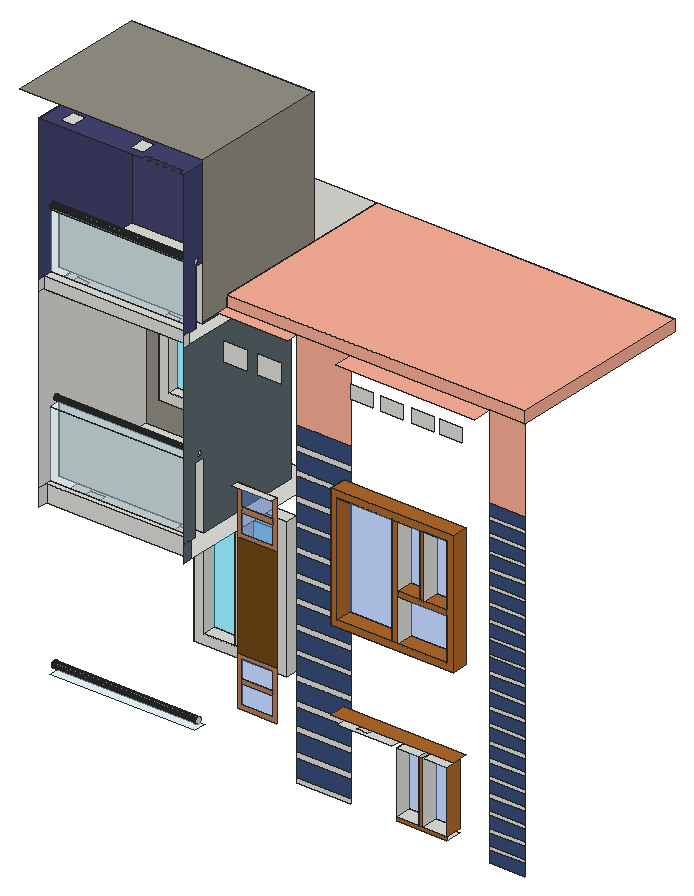
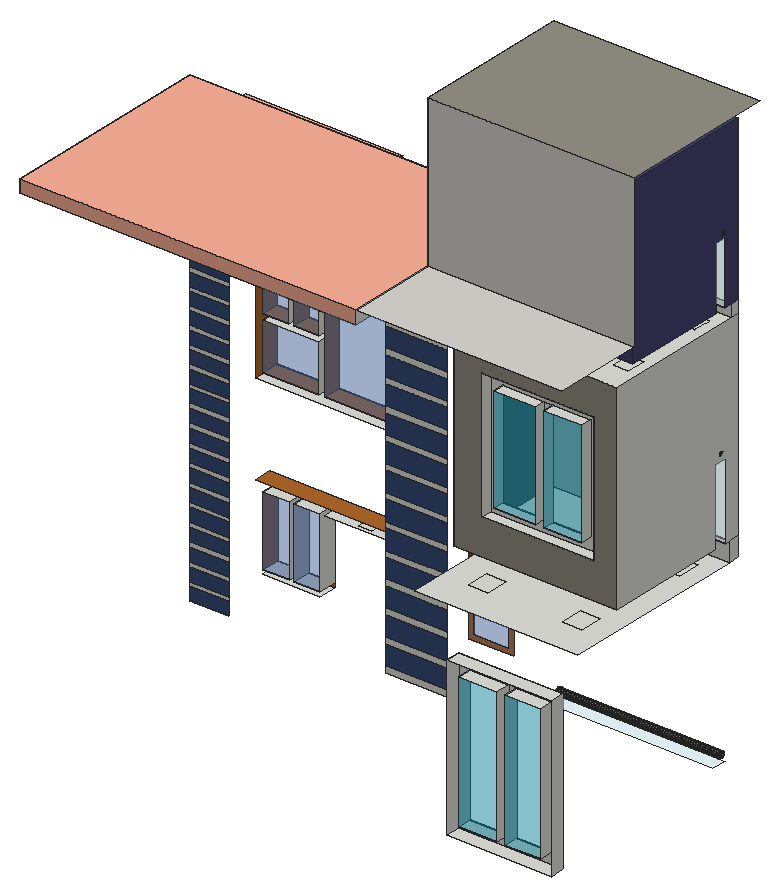
# SketchUp Ruby script. Lengths in inches.
U = 1.inch
M = Sketchup.active_model
def pt(a) = Geom::Point3d.new(a.map { |v| v * U })
def face(e, loops, mat)
  f = e.add_face(loops[0].map { |a| pt(a) })
  loops[1..].each { |l| e.add_face(l.map { |a| pt(a) }).erase! }
  f.material = f.back_material = mat if mat
  f
end
# faces: each face lists its corners as indices into pts; further lists are holes
def faces(e, pts, list, mat = nil) = list.each { |f| face(e, (f[0].is_a?(Array) ? f : [f]).map { |l| l.map { |i| pts[i] } }, mat) }
# xy, xz, yz: faces in a plane at the given z, y or x. An outline is a flat list of corners, or four numbers for a rectangle; further outlines are holes
def ring(l) = l.size == 4 ? [[l[0], l[1]], [l[2], l[1]], [l[2], l[3]], [l[0], l[3]]] : l.each_slice(2).to_a
def flat(e, list, mat, &to3) = list.each { |f| face(e, (f[0].is_a?(Array) ? f : [f]).map { |l| ring(l).map { |u, v| to3.(u, v) } }, mat) }
def xy(e, z, list, mat = nil) = flat(e, list, mat) { |x, y| [x, y, z] }
def xz(e, y, list, mat = nil) = flat(e, list, mat) { |x, z| [x, y, z] }
def yz(e, x, list, mat = nil) = flat(e, list, mat) { |y, z| [x, y, z] }
def lines(e, pts, list) = list.each { |a, b| e.add_line(pt(pts[a]), pt(pts[b])) }
# prism: a flat outline (further loops are holes) pulled along v
def prism(e, loops, v, mat = nil)
  f = face(e, loops, mat); d = Geom::Vector3d.new(v.map { |x| x * U })
  f.pushpull(f.normal.samedirection?(d) ? d.length : -d.length)
end
def box(e, o, s, mat = nil) = prism(e, [[o, [o[0] + s[0], o[1], o[2]], [o[0] + s[0], o[1] + s[1], o[2]], [o[0], o[1] + s[1], o[2]]]], [0, 0, s[2]], mat)
def at(x, y, z, deg = 0) = Geom::Transformation.translation(pt([x, y, z])) * Geom::Transformation.rotation(ORIGIN, Z_AXIS, deg.degrees)
def axes(o, x, y, z) = Geom::Transformation.new([*x, 0, *y, 0, *z, 0, *pt(o).to_a, 1])
def part(name) = M.definitions.add(name)
# library, detail: a bought-in or finely detailed component or shape, given as its bounding box
def library(name, o, s) = part(name).tap { |d| box(d.entities, o, s) }
def detail(e, o, s) = box(e.add_group.entities, o, s)
def put(e, d, t, mat = nil) = e.add_instance(d, t).tap { |i| i.material = mat if mat }
def group(e, t, mat = nil) = e.add_group.tap { |g| g.transformation = t; g.material = mat if mat }.entities
root = M.entities
M.materials.add("[Blinds Weave]").color = [114, 74, 20]
M.materials.add("[Color B02]").color = [255, 178, 153]
M.materials.add("[Color I02]").color = [68, 68, 114]
M.materials.add("[Formica Blue]").color = [58, 79, 124]
M.materials.add("[Formica Graystone]").color = [149, 146, 135]
M.materials.add("[Formica Speckled Grey]").color = [94, 105, 111]
M.materials.add("[Terrazzo Tile Light]").color = [219, 217, 210]
M.materials.add("[Translucent Glass Blue]").color = [100, 149, 237]
M.materials["[Translucent Glass Blue]"].alpha = 0.5
M.materials.add("[Translucent Glass Safety]").color = [204, 235, 244]
M.materials["[Translucent Glass Safety]"].alpha = 0.5
M.materials.add("[Translucent Glass Tinted]").color = [8, 201, 241]
M.materials["[Translucent Glass Tinted]"].alpha = 0.48
M.materials.add("[Wood Bamboo]").color = [177, 105, 43]
M.materials.add("[Wood Veneer 02]").color = [190, 128, 91]
xy(root,1117.04,[[74.41,296.125,237.41,318.5]])
xy(root,1134.79,[[92.16,296.125,146.9375,318.5],[159.55,296.125,219.66,318.5]])
xy(root,1165.4,[[33.32,31.52,287.32,55.75]],"[Translucent Glass Safety]")
xy(root,1171.56,[[667.45,0,756.11,28.0625]])
xy(root,1178.11,[[667.45,0,707.8,28.0625],[714.14,0,756.11,28.0625]])
xy(root,1286.6,[[[564.0625,0,660.09,28.0625],[592.18,6.79,612.12,21.73]],[667.45,0,707.8,28.0625],[714.14,0,756.11,28.0625],[592.18,6.79,612.12,21.73]])
xy(root,1298.36,[[552.31,0,767.87,28.0625]],"[Wood Bamboo]")
xy(root,1344.23,[[92.16,296.125,146.9375,318.5],[159.55,296.125,219.66,318.5]])
xy(root,1361.98,[[74.41,296.125,237.41,318.5]])
xy(root,1439.76,[[[33.32,24,287.32,318.5],[59.3,52.79,88.73,87.54],[216.42,52.79,245.86,87.54],[216.42,230.73,245.86,265.48],[69.67,230.73,99.11,265.48]],[59.3,52.79,88.73,87.54],[216.42,52.79,245.86,87.54],[69.67,230.73,99.11,265.48],[216.42,230.73,245.86,265.48]])
xy(root,1440.48,[[552.31,0,767.87,28.0625]])
xy(root,1451.8,[[563.625,0,660.09,28.0625],[669.72,0,756.55,28.0625]],"[Wood Bamboo]")
xy(root,1469.71,[[33.32,24,287.32,31.88],[33.32,51.68,287.32,242.375]])
xy(root,1525.5,[[69.375,225.25,243.875,242.375]])
xy(root,1525.64,[[669.72,0,756.55,28.0625]])
xy(root,1534.53,[[669.72,0,707.93,28.0625],[716.55,0,756.55,28.0625]],"[Wood Bamboo]")
xy(root,1544.08,[[87.96,225.25,147.05,242.375],[160.71,225.25,225.3,242.375]])
xy(root,1568.875,[[345.55,40.625,414.87,53.5625]])
xy(root,1587.65,[[33.32,31.88,287.32,51.68]],"[Translucent Glass Safety]")
xy(root,1644.72,[[[563.625,0,660.09,28.0625],[594.73,5.47,608.73,22.59]],[669.72,0,707.93,28.0625],[716.55,0,756.55,28.0625],[594.73,5.47,608.73,22.59]])
xy(root,1656.05,[[552.31,0,767.87,28.0625]],"[Wood Bamboo]")
xy(root,1707.74,[[87.96,225.25,147.05,242.375],[160.71,225.25,225.3,242.375]])
xy(root,1726.32,[[69.375,225.25,243.875,242.375]])
xy(root,1779.22,[[[33.32,18.6875,287.32,242.375],[49.04,41.2,72.04,71.89],[49.04,171.01,72.04,201.7],[210.73,41.2,233.73,71.89],[210.73,175.64,233.73,206.32]],[49.04,41.2,72.04,71.89],[210.73,41.2,233.73,71.89],[49.04,171.01,72.04,201.7],[210.73,175.64,233.73,206.32]])
xy(root,1798.56,[[33.32,18.6875,287.32,33.35],[33.32,50.86,287.32,211.6875]])
xy(root,1831.875,[[320.63,61.625,843.32,391.54]])
xy(root,1831.875,[[538.37,28.0625,782.27,61.625],[320.63,40.625,443.82,61.625]],"[Color B02]")
xy(root,1852.125,[[320.63,61.625,843.32,391.54]],"[Color B02]")
xy(root,1852.125,[[0,252.1,320.63,391.54]],"[Terrazzo Tile Light]")
xy(root,1896.06,[[33.32,33.35,287.32,50.86]],"[Translucent Glass Safety]")
xy(root,2052.75,[[61.875,22.48,80.9375,48.04],[183.75,22.48,202.8125,48.04]])
xy(root,2052.75,[[[33.32,7.5,33.32,211.6875,287.32,211.6875,287.32,7.5,280.35,7.5,280.35,17.375,269.11,17.375,269.11,7.5,266.35,7.5,266.35,17.375,255.11,17.375,255.11,7.5,252.29,7.5,252.29,17.375,241.05,17.375,241.05,7.5,238.35,7.5,238.35,17.375,227.11,17.375,227.11,7.5,224.6,7.5,224.6,17.375,213.36,17.375,213.36,7.5],[61.875,22.48,80.9375,48.04],[183.75,22.48,202.8125,48.04]]],"[Color I02]")
xy(root,2087.5625,[[0,7.5,320.63,252.1]],"[Formica Graystone]")
xz(root,0,[[667.45,1171.56,756.11,1178.11],[707.8,1178.11,714.14,1286.6],[[552.31,1440.48,767.87,1656.05],[563.625,1451.8,756.55,1644.72]],[660.09,1451.8,669.72,1644.72],[669.72,1525.64,756.55,1534.53],
  [707.93,1534.53,716.55,1644.72]],"[Wood Bamboo]")
xz(root,18.6875,[[33.32,1779.22,287.32,1798.56]])
xz(root,24,[[33.32,1439.76,287.32,1469.71]])
xz(root,28.0625,[[565.47,1787.53,604,1811.34],[618.59,1787.53,657.12,1811.34],[671.78,1787.53,710.31,1811.34],[721.9,1787.53,760.43,1811.34]])
xz(root,28.0625,[[667.45,1178.11,707.8,1286.6],[714.14,1178.11,756.11,1286.6],[563.625,1451.8,660.09,1644.72],[669.72,1451.8,756.55,1525.64],[669.72,1534.53,707.93,1644.72],
  [716.55,1534.53,756.55,1644.72]],"[Translucent Glass Blue]")
xz(root,31.88,[[33.32,1469.71,287.32,1587.65]],"[Translucent Glass Safety]")
xz(root,33.35,[[33.32,1798.56,287.32,1896.06]],"[Translucent Glass Safety]")
xz(root,40.625,[[331.73,1759.52,372.85,1792.7],[390.85,1759.52,431.98,1792.7]])
xz(root,50.86,[[33.32,1798.56,287.32,1896.06]])
xz(root,51.68,[[33.32,1469.71,287.32,1587.65]])
xz(root,53.5625,[[345.55,1299.8,414.87,1482.92]],"[Blinds Weave]")
xz(root,53.5625,[[353.125,1220.24,407.29,1253.6875],[353.125,1262.02,407.29,1292.22],[352.96,1490.32,407.46,1522.55],[352.96,1532.46,407.46,1561.47]],"[Translucent Glass Blue]")
xz(root,53.5625,[[[345.55,1212.67,414.87,1299.8],[353.125,1220.24,407.29,1292.22]],[353.125,1253.6875,407.29,1262.02],[[345.55,1482.92,414.87,1568.875],[352.96,1490.32,407.46,1561.47]],[352.96,1522.55,407.46,1532.46]],"[Wood Veneer 02]")
xz(root,61.625,[[443.82,1125.38,538.37,1134.51],[782.27,1139.9375,843.32,1145.125],[443.82,1165.69,538.37,1174.82],[782.27,1166.1875,843.32,1172.8125],[782.27,1193.875,843.32,1200.5],
  [443.82,1206.01,538.37,1215.13],[782.27,1221.5625,843.32,1228.1875],[443.82,1246.32,538.37,1255.44],[782.27,1249.25,843.32,1255.875],[782.27,1276.9375,843.32,1283.5625],
  [443.82,1286.63,538.37,1295.76],[782.27,1304.625,843.32,1311.25],[443.82,1326.94,538.37,1336.07],[782.27,1332.3125,843.32,1338.9375],[782.27,1360,843.32,1366.625],
  [443.82,1367.26,538.37,1376.38],[782.27,1387.6875,843.32,1394.3125],[443.82,1407.57,538.37,1416.69],[782.27,1415.375,843.32,1421.375],[782.27,1442.4375,843.32,1448.4375],
  [443.82,1447.88,538.37,1457.01],[782.27,1469.5,843.32,1475.5],[443.82,1488.19,538.37,1497.32],[782.27,1496.5625,843.32,1502.5625],[782.27,1523.625,843.32,1529.625],
  [443.82,1528.51,538.37,1537.63],[782.27,1550.6875,843.32,1556.6875],[443.82,1568.82,538.37,1577.94],[782.27,1577.75,843.32,1583.75],[782.27,1604.8125,843.32,1610.8125],
  [443.82,1609.13,538.37,1618.26],[782.27,1631.875,843.32,1637.875],[443.82,1649.44,538.37,1658.57],[782.27,1658.9375,843.32,1664.9375]])
xz(root,61.625,[[782.27,1686,843.32,1831.875],[443.82,1689.76,538.37,1831.875],[320.63,1831.875,843.32,1852.125]],"[Color B02]")
xz(root,61.625,[[782.27,1118.875,843.32,1139.9375],[443.82,1134.51,538.37,1165.69],[782.27,1145.125,843.32,1166.1875],[782.27,1172.8125,843.32,1193.875],[443.82,1174.82,538.37,1206.01],
  [782.27,1200.5,843.32,1221.5625],[443.82,1215.13,538.37,1246.32],[782.27,1228.1875,843.32,1249.25],[443.82,1255.44,538.37,1286.63],[782.27,1255.875,843.32,1276.9375],
  [782.27,1283.5625,843.32,1304.625],[443.82,1295.76,538.37,1326.94],[782.27,1311.25,843.32,1332.3125],[443.82,1336.07,538.37,1367.26],[782.27,1338.9375,843.32,1360],
  [782.27,1366.625,843.32,1387.6875],[443.82,1376.38,538.37,1407.57],[782.27,1394.3125,843.32,1415.375],[443.82,1416.69,538.37,1447.88],[782.27,1421.375,843.32,1442.4375],
  [782.27,1448.4375,843.32,1469.5],[443.82,1457.01,538.37,1488.19],[782.27,1475.5,843.32,1496.5625],[443.82,1497.32,538.37,1528.51],[782.27,1502.5625,843.32,1523.625],
  [782.27,1529.625,843.32,1550.6875],[443.82,1537.63,538.37,1568.82],[782.27,1556.6875,843.32,1577.75],[443.82,1577.94,538.37,1609.13],[782.27,1583.75,843.32,1604.8125],
  [782.27,1610.8125,843.32,1631.875],[443.82,1618.26,538.37,1649.44],[782.27,1637.875,843.32,1658.9375],[443.82,1658.57,538.37,1689.76],[782.27,1664.9375,843.32,1686]],"[Formica Blue]")
xz(root,211.6875,[[33.32,1798.56,287.32,2052.75]],"[Color I02]")
xz(root,225.25,[[[69.375,1525.5,243.875,1726.32],[87.96,1544.08,225.3,1707.74]],[147.05,1544.08,160.71,1707.74]])
xz(root,242.375,[[[33.32,1469.71,287.32,1779.22],[69.375,1525.5,243.875,1726.32]]],"[Formica Graystone]")
xz(root,242.375,[[87.96,1544.08,147.05,1707.74],[160.71,1544.08,225.3,1707.74]],"[Translucent Glass Tinted]")
xz(root,252.1,[[0,1852.125,320.63,2087.5625]],"[Terrazzo Tile Light]")
xz(root,296.125,[[[74.41,1117.04,237.41,1361.98],[92.16,1134.79,219.66,1344.23]],[146.9375,1134.79,159.55,1344.23]])
xz(root,318.5,[[92.16,1134.79,146.9375,1344.23],[159.55,1134.79,219.66,1344.23]],"[Translucent Glass Tinted]")
xz(root,391.54,[[320.63,1831.875,843.32,1852.125]],"[Color B02]")
yz(root,33.32,[[7.5,1439.76,24,1469.71],[[7.5,1469.71,31.88,1469.71,31.88,1587.65,51.68,1587.65,51.68,1469.71,242.375,1469.71,242.375,1779.22,7.5,1779.22],[41.78,1594.54,40.73,1594.68,39.76,1595.09,38.92,1595.73,38.28,1596.57,37.875,1597.54,37.74,1598.59,37.875,1599.64,38.28,1600.61,38.92,1601.45,39.76,1602.09,40.73,1602.5,41.78,1602.63,42.83,1602.5,43.8,1602.09,44.64,1601.45,45.28,1600.61,45.6875,1599.64,45.83,1598.59,45.6875,1597.54,45.28,1596.57,44.64,1595.73,43.8,1595.09,42.83,1594.68]],[7.5,1779.22,18.6875,1798.56]])
yz(root,33.32,[[[7.5,1798.56,33.35,1798.56,33.35,1896.06,50.86,1896.06,50.86,1798.56,211.6875,1798.56,211.6875,2052.75,7.5,2052.75],[34.6,1899.44,33.32,1899.61,32.125,1900.1,31.1,1900.89,30.32,1901.91,29.83,1903.1,29.66,1904.38,29.83,1905.66,30.32,1906.85,31.1,1907.87,32.125,1908.66,33.32,1909.15,34.6,1909.32,35.875,1909.15,37.0625,1908.66,38.09,1907.87,38.87,1906.85,39.36,1905.66,39.53,1904.38,39.36,1903.1,38.87,1901.91,38.09,1900.89,37.0625,1900.1,35.875,1899.61]]],"[Color I02]")
yz(root,69.375,[[225.25,1525.5,242.375,1726.32]])
yz(root,74.41,[[296.125,1117.04,318.5,1361.98]])
yz(root,87.96,[[225.25,1544.08,242.375,1707.74]])
yz(root,92.16,[[296.125,1134.79,318.5,1344.23]])
yz(root,146.9375,[[296.125,1134.79,318.5,1344.23]])
yz(root,147.05,[[225.25,1544.08,242.375,1707.74]])
yz(root,159.55,[[296.125,1134.79,318.5,1344.23]])
yz(root,160.71,[[225.25,1544.08,242.375,1707.74]])
yz(root,219.66,[[296.125,1134.79,318.5,1344.23]])
yz(root,225.3,[[225.25,1544.08,242.375,1707.74]])
yz(root,237.41,[[296.125,1117.04,318.5,1361.98]])
yz(root,243.875,[[225.25,1525.5,242.375,1726.32]])
yz(root,287.32,[[40.12,1173.19,41.49,1173.37,42.77,1173.9,43.875,1174.75,44.72,1175.85,45.25,1177.13,45.43,1178.5,45.25,1179.88,44.72,1181.16,43.875,1182.26,42.77,1183.1,41.49,1183.63,40.12,1183.82,38.74,1183.63,37.46,1183.1,36.36,1182.26,35.52,1181.16,34.99,1179.88,34.81,1178.5,34.99,1177.13,35.52,1175.85,36.36,1174.75,37.46,1173.9,38.74,1173.37],[41.78,1594.54,42.83,1594.68,43.8,1595.09,44.64,1595.73,45.28,1596.57,45.6875,1597.54,45.83,1598.59,45.6875,1599.64,45.28,1600.61,44.64,1601.45,43.8,1602.09,42.83,1602.5,41.78,1602.63,40.73,1602.5,39.76,1602.09,38.92,1601.45,38.28,1600.61,37.875,1599.64,37.74,1598.59,37.875,1597.54,38.28,1596.57,38.92,1595.73,39.76,1595.09,40.73,1594.68],[7.5,1779.22,18.6875,1798.56],[34.6,1899.44,35.875,1899.61,37.0625,1900.1,38.09,1900.89,38.87,1901.91,39.36,1903.1,39.53,1904.38,39.36,1905.66,38.87,1906.85,38.09,1907.87,37.0625,1908.66,35.875,1909.15,34.6,1909.32,33.32,1909.15,32.125,1908.66,31.1,1907.87,30.32,1906.85,29.83,1905.66,29.66,1904.38,29.83,1903.1,30.32,1901.91,31.1,1900.89,32.125,1900.1,33.32,1899.61]])
yz(root,287.32,[[[7.5,1798.56,7.5,2052.75,211.6875,2052.75,211.6875,1798.56,50.86,1798.56,50.86,1896.06,33.35,1896.06,33.35,1798.56],[34.6,1899.44,35.875,1899.61,37.0625,1900.1,38.09,1900.89,38.87,1901.91,39.36,1903.1,39.53,1904.38,39.36,1905.66,38.87,1906.85,38.09,1907.87,37.0625,1908.66,35.875,1909.15,34.6,1909.32,33.32,1909.15,32.125,1908.66,31.1,1907.87,30.32,1906.85,29.83,1905.66,29.66,1904.38,29.83,1903.1,30.32,1901.91,31.1,1900.89,32.125,1900.1,33.32,1899.61]]],"[Color I02]")
yz(root,287.32,[[7.5,1439.76,24,1469.71],[[7.5,1469.71,7.5,1779.22,242.375,1779.22,242.375,1469.71,51.68,1469.71,51.68,1587.65,31.88,1587.65,31.88,1469.71],[41.78,1594.54,42.83,1594.68,43.8,1595.09,44.64,1595.73,45.28,1596.57,45.6875,1597.54,45.83,1598.59,45.6875,1599.64,45.28,1600.61,44.64,1601.45,43.8,1602.09,42.83,1602.5,41.78,1602.63,40.73,1602.5,39.76,1602.09,38.92,1601.45,38.28,1600.61,37.875,1599.64,37.74,1598.59,37.875,1597.54,38.28,1596.57,38.92,1595.73,39.76,1595.09,40.73,1594.68]]],"[Formica Speckled Grey]")
yz(root,320.63,[[61.625,1831.875,391.54,1852.125]])
yz(root,320.63,[[7.5,1831.875,61.625,1831.875,61.625,1852.125,252.1,1852.125,252.1,2087.5625,7.5,2087.5625]],"[Formica Graystone]")
yz(root,552.31,[[0,1440.48,28.0625,1656.05]],"[Wood Bamboo]")
yz(root,563.625,[[0,1451.8,28.0625,1644.72]],"[Wood Bamboo]")
yz(root,660.09,[[0,1451.8,28.0625,1644.72]],"[Wood Bamboo]")
yz(root,667.45,[[0,1178.11,28.0625,1286.6]])
yz(root,669.72,[[0,1451.8,28.0625,1525.64],[0,1534.53,28.0625,1644.72]])
yz(root,707.8,[[0,1178.11,28.0625,1286.6]])
yz(root,707.93,[[0,1534.53,28.0625,1644.72]],"[Wood Bamboo]")
yz(root,714.14,[[0,1178.11,28.0625,1286.6]])
yz(root,716.55,[[0,1534.53,28.0625,1644.72]])
yz(root,756.11,[[0,1178.11,28.0625,1286.6]],"[Wood Bamboo]")
yz(root,756.55,[[0,1451.8,28.0625,1525.64],[0,1534.53,28.0625,1644.72]],"[Wood Bamboo]")
yz(root,767.87,[[0,1440.48,28.0625,1656.05]],"[Wood Bamboo]")
yz(root,843.32,[[61.625,1831.875,391.54,1852.125]],"[Color B02]")
p = [[287.32,40.12,1173.19],[287.32,38.74,1173.37],[33.32,38.74,1173.37],[33.32,40.12,1173.19],[287.32,41.49,1173.37],[33.32,41.49,1173.37],
  [287.32,37.46,1173.9],[33.32,37.46,1173.9],[287.32,42.77,1173.9],[33.32,42.77,1173.9],[287.32,36.36,1174.75],[33.32,36.36,1174.75],
  [287.32,43.875,1174.75],[33.32,43.875,1174.75],[287.32,35.52,1175.85],[33.32,35.52,1175.85],[287.32,44.72,1175.85],[33.32,44.72,1175.85],
  [287.32,34.99,1177.13],[33.32,34.99,1177.13],[287.32,45.25,1177.13],[33.32,45.25,1177.13],[287.32,34.81,1178.5],[33.32,34.81,1178.5],
  [287.32,45.43,1178.5],[33.32,45.43,1178.5],[287.32,34.99,1179.88],[33.32,34.99,1179.88],[287.32,45.25,1179.88],[33.32,45.25,1179.88],
  [287.32,35.52,1181.16],[33.32,35.52,1181.16],[287.32,44.72,1181.16],[33.32,44.72,1181.16],[287.32,36.36,1182.26],[33.32,36.36,1182.26],
  [287.32,43.875,1182.26],[33.32,43.875,1182.26],[287.32,37.46,1183.1],[33.32,37.46,1183.1],[287.32,42.77,1183.1],[33.32,42.77,1183.1],
  [287.32,38.74,1183.63],[33.32,38.74,1183.63],[287.32,41.49,1183.63],[33.32,41.49,1183.63],[287.32,40.12,1183.82],[33.32,40.12,1183.82],
  [287.32,41.78,1594.54],[287.32,40.73,1594.68],[33.32,40.73,1594.68],[33.32,41.78,1594.54],[287.32,42.83,1594.68],[33.32,42.83,1594.68],
  [287.32,39.76,1595.09],[33.32,39.76,1595.09],[287.32,43.8,1595.09],[33.32,43.8,1595.09],[287.32,38.92,1595.73],[33.32,38.92,1595.73],
  [287.32,44.64,1595.73],[33.32,44.64,1595.73],[287.32,38.28,1596.57],[33.32,38.28,1596.57],[287.32,45.28,1596.57],[33.32,45.28,1596.57],
  [287.32,37.875,1597.54],[33.32,37.875,1597.54],[287.32,45.6875,1597.54],[33.32,45.6875,1597.54],[287.32,37.74,1598.59],[33.32,37.74,1598.59],
  [287.32,45.83,1598.59],[33.32,45.83,1598.59],[287.32,37.875,1599.64],[33.32,37.875,1599.64],[287.32,45.6875,1599.64],[33.32,45.6875,1599.64],
  [287.32,38.28,1600.61],[33.32,38.28,1600.61],[287.32,45.28,1600.61],[33.32,45.28,1600.61],[287.32,38.92,1601.45],[33.32,38.92,1601.45],
  [287.32,44.64,1601.45],[33.32,44.64,1601.45],[287.32,39.76,1602.09],[33.32,39.76,1602.09],[287.32,43.8,1602.09],[33.32,43.8,1602.09],
  [287.32,40.73,1602.5],[33.32,40.73,1602.5],[287.32,42.83,1602.5],[33.32,42.83,1602.5],[287.32,41.78,1602.63],[33.32,41.78,1602.63],
  [287.32,34.6,1899.44],[287.32,33.32,1899.61],[33.32,33.32,1899.61],[33.32,34.6,1899.44],[287.32,35.875,1899.61],[33.32,35.875,1899.61],
  [287.32,32.125,1900.1],[33.32,32.125,1900.1],[287.32,37.0625,1900.1],[33.32,37.0625,1900.1],[287.32,31.1,1900.89],[33.32,31.1,1900.89],
  [287.32,38.09,1900.89],[33.32,38.09,1900.89],[287.32,30.32,1901.91],[33.32,30.32,1901.91],[287.32,38.87,1901.91],[33.32,38.87,1901.91],
  [287.32,29.83,1903.1],[33.32,29.83,1903.1],[287.32,39.36,1903.1],[33.32,39.36,1903.1],[287.32,29.66,1904.38],[33.32,29.66,1904.38],
  [287.32,39.53,1904.38],[33.32,39.53,1904.38],[287.32,29.83,1905.66],[33.32,29.83,1905.66],[287.32,39.36,1905.66],[33.32,39.36,1905.66],
  [287.32,30.32,1906.85],[33.32,30.32,1906.85],[287.32,38.87,1906.85],[33.32,38.87,1906.85],[287.32,31.1,1907.87],[33.32,31.1,1907.87],
  [287.32,38.09,1907.87],[33.32,38.09,1907.87],[287.32,32.125,1908.66],[33.32,32.125,1908.66],[287.32,37.0625,1908.66],[33.32,37.0625,1908.66],
  [287.32,33.32,1909.15],[33.32,33.32,1909.15],[287.32,35.875,1909.15],[33.32,35.875,1909.15],[287.32,34.6,1909.32],[33.32,34.6,1909.32]]
faces(root,p,[[0,1,2,3],[4,0,3,5],[1,6,7,2],[8,4,5,9],[6,10,11,7],[12,8,9,13],[10,14,15,11],[16,12,13,17],
  [14,18,19,15],[20,16,17,21],[18,22,23,19],[24,20,21,25],[22,26,27,23],[28,24,25,29],[26,30,31,27],[32,28,29,33],
  [30,34,35,31],[36,32,33,37],[34,38,39,35],[40,36,37,41],[38,42,43,39],[44,40,41,45],[42,46,47,43],[46,44,45,47],
  [48,49,50,51],[52,48,51,53],[49,54,55,50],[56,52,53,57],[54,58,59,55],[60,56,57,61],[58,62,63,59],[64,60,61,65],
  [62,66,67,63],[68,64,65,69],[66,70,71,67],[72,68,69,73],[70,74,75,71],[76,72,73,77],[74,78,79,75],[80,76,77,81],
  [78,82,83,79],[84,80,81,85],[82,86,87,83],[88,84,85,89],[86,90,91,87],[92,88,89,93],[90,94,95,91],[94,92,93,95],
  [96,97,98,99],[100,96,99,101],[97,102,103,98],[104,100,101,105],[102,106,107,103],[108,104,105,109],[106,110,111,107],[112,108,109,113],
  [110,114,115,111],[116,112,113,117],[114,118,119,115],[120,116,117,121],[118,122,123,119],[124,120,121,125],[122,126,127,123],[128,124,125,129],
  [126,130,131,127],[132,128,129,133],[130,134,135,131],[136,132,133,137],[134,138,139,135],[140,136,137,141],[138,142,143,139],[142,140,141,143]],"[Formica Graystone]")
